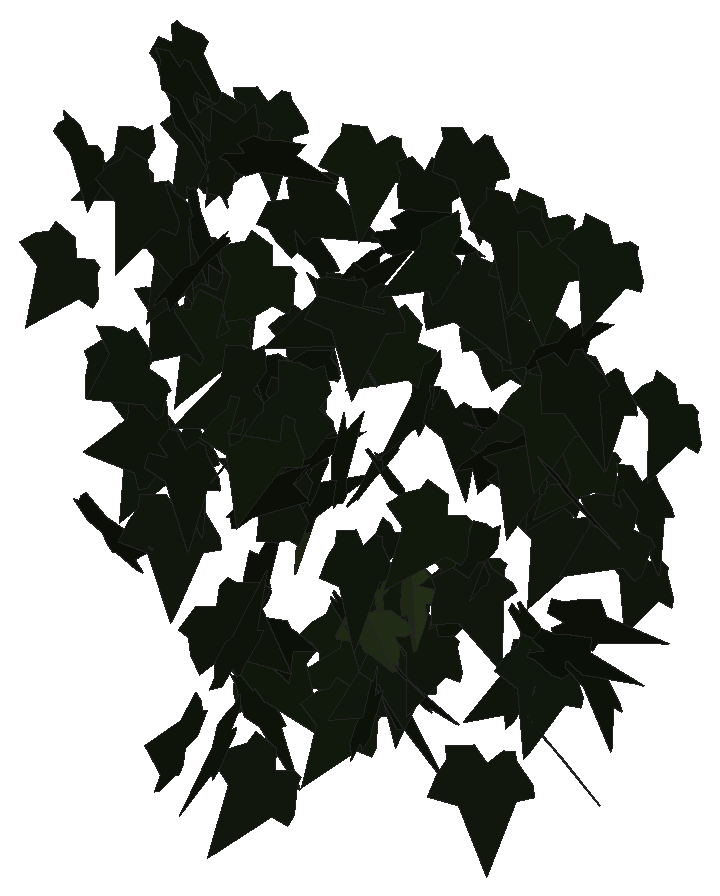
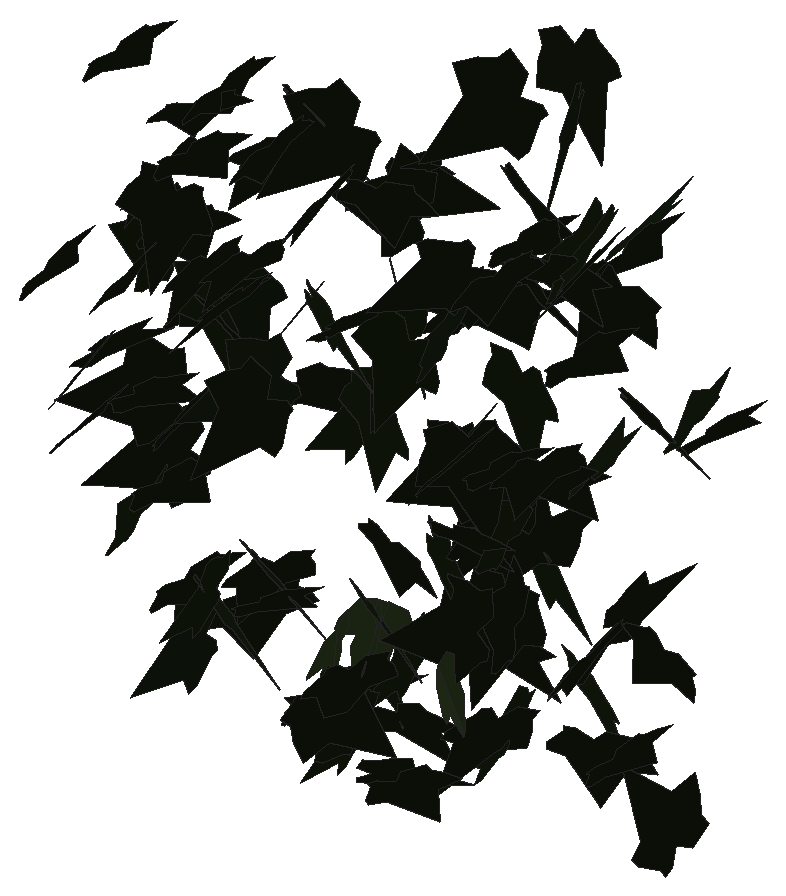
# SketchUp Ruby script. Lengths in inches.
U = 1.inch
M = Sketchup.active_model
def pt(a) = Geom::Point3d.new(a.map { |v| v * U })
def face(e, loops, mat)
  f = e.add_face(loops[0].map { |a| pt(a) })
  loops[1..].each { |l| e.add_face(l.map { |a| pt(a) }).erase! }
  f.material = f.back_material = mat if mat
  f
end
# faces: each face lists its corners as indices into pts; further lists are holes
def faces(e, pts, list, mat = nil) = list.each { |f| face(e, (f[0].is_a?(Array) ? f : [f]).map { |l| l.map { |i| pts[i] } }, mat) }
# xy, xz, yz: faces in a plane at the given z, y or x. An outline is a flat list of corners, or four numbers for a rectangle; further outlines are holes
def ring(l) = l.size == 4 ? [[l[0], l[1]], [l[2], l[1]], [l[2], l[3]], [l[0], l[3]]] : l.each_slice(2).to_a
def flat(e, list, mat, &to3) = list.each { |f| face(e, (f[0].is_a?(Array) ? f : [f]).map { |l| ring(l).map { |u, v| to3.(u, v) } }, mat) }
def xy(e, z, list, mat = nil) = flat(e, list, mat) { |x, y| [x, y, z] }
def xz(e, y, list, mat = nil) = flat(e, list, mat) { |x, z| [x, y, z] }
def yz(e, x, list, mat = nil) = flat(e, list, mat) { |y, z| [x, y, z] }
def lines(e, pts, list) = list.each { |a, b| e.add_line(pt(pts[a]), pt(pts[b])) }
# prism: a flat outline (further loops are holes) pulled along v
def prism(e, loops, v, mat = nil)
  f = face(e, loops, mat); d = Geom::Vector3d.new(v.map { |x| x * U })
  f.pushpull(f.normal.samedirection?(d) ? d.length : -d.length)
end
def box(e, o, s, mat = nil) = prism(e, [[o, [o[0] + s[0], o[1], o[2]], [o[0] + s[0], o[1] + s[1], o[2]], [o[0], o[1] + s[1], o[2]]]], [0, 0, s[2]], mat)
def at(x, y, z, deg = 0) = Geom::Transformation.translation(pt([x, y, z])) * Geom::Transformation.rotation(ORIGIN, Z_AXIS, deg.degrees)
def axes(o, x, y, z) = Geom::Transformation.new([*x, 0, *y, 0, *z, 0, *pt(o).to_a, 1])
def part(name) = M.definitions.add(name)
# library, detail: a bought-in or finely detailed component or shape, given as its bounding box
def library(name, o, s) = part(name).tap { |d| box(d.entities, o, s) }
def detail(e, o, s) = box(e.add_group.entities, o, s)
def put(e, d, t, mat = nil) = e.add_instance(d, t).tap { |i| i.material = mat if mat }
def group(e, t, mat = nil) = e.add_group.tap { |g| g.transformation = t; g.material = mat if mat }.entities
root = M.entities
M.materials.add("efeu1").color = [18, 25, 13]
M.materials.add("efeu2").color = [43, 57, 29]
c1 = part("ivyleaf_9")
p = [[1.54,2.16,1.25],[1.36,2.04,1.19],[-0.21,0.99,0.68],[-0.71,1.11,0.82],[-0.85,0.86,0.67],[-0.8,0.17,0.21],
  [-0.9,-0.01,0.1],[-0.67,-0.16,-0.02],[-0.08,-0.08,-0.05],[-0.03,-0.6,-0.4],[0.65,-0.88,-0.66],[0.83,-0.6,-0.49],
  [1.29,-0.42,-0.43],[1.8125,-0.07,-0.26],[1.21,0.44,0.15]]
faces(c1.entities,p,[[0,1,2,3,4,5,6,7,8,9,10,11,12,13,14]],"efeu1")
c2 = part("ivyleaf_10")
p = [[0,0.5,-0.03],[-0.0625,2.02,-0.43],[-0.19,2.01,-0.46],[-0.54,1.05,-0.29],[-0.52,0.625,-0.18],[-0.83,0.76,-0.28],
  [-1.16,0.64,-0.33],[-1.15,0.33,-0.24],[-0.77,-0.39,0.02],[-0.3,-0.51,0.16],[0.04,-0.48,0.23],[-0.02,2.01,-0.4375],
  [-0.06,2.01,-0.43],[0.04,-0.49,0.23],[0.67,-0.49,0.14],[1.38,0.36,-0.2],[1.375,0.51,-0.24],[0.81,0.65,-0.19],
  [0.62,0.59,-0.15],[0.6,1.09,-0.28],[0.5,1.23,-0.31]]
faces(c2.entities,p,[[0,1,2,3,4,5,6,7,8,9,10],[11,12,0,13,14,15,16,17,18,19,20]],"efeu2")
put(root,c1,axes([587.55,109.1,321.87],[-0.72826,-0.69552,1.1133],[-0.03534,-1.2623,-0.81172],[1.31223,-0.42,0.596]))
put(root,c1,axes([592.26,108.54,307.04],[-1.13952,0.73613,-0.62099],[0.53113,-0.32215,-1.35651],[-0.80338,-1.25712,-0.01601]))
put(root,c1,axes([590.89,108.03,328.35],[-0.38313,1.43362,-0.19459],[0.05066,-0.18788,-1.48393],[-1.44588,-0.38646,-0.00043]))
put(root,c1,axes([592.6,110.86,304.26],[-1.38279,-0.46875,-0.09816],[0.09636,0.02149,-1.46004],[0.46912,-1.3861,0.01056]))
put(root,c1,axes([591.54,109.78,309.39],[-0.99939,0.98729,-0.32059],[-0.27455,0.17776,1.40332],[1.00107,1.03439,0.06482]))
put(root,c1,axes([588.24,110.67,303.98],[-0.75989,1.06786,0.64427],[-0.34194,0.54714,-1.31017],[-1.19937,-0.83256,-0.03466]))
put(root,c1,axes([591.34,111.97,319.29],[-0.7287,-1.23215,-0.15341],[0.08749,0.12649,-1.43147],[1.23858,-0.73386,0.01085]))
put(root,c1,axes([588.37,111.2,328.16],[0.83103,-0.28067,-1.21153],[-1.10919,0.49166,-0.87473],[0.56239,1.38445,0.06503]))
put(root,c1,axes([590.68,111.88,320.77],[-1.35145,0.54253,0.34301],[-0.31812,0.12828,-1.45628],[-0.55748,-1.38838,-0.00051]))
put(root,c1,axes([589.53,111.39,310.48],[0.18456,-0.60274,-1.36473],[-0.14342,1.3616,-0.62075],[1.485,0.20641,0.10966]))
put(root,c1,axes([592.26,114.1,319.52],[-0.63385,-0.52593,1.13026],[-0.77577,-0.82614,-0.81947],[0.97584,-0.99837,0.08269]))
put(root,c1,axes([593.95,114.74,324.5],[-0.18122,-0.22106,-1.38757],[-0.20509,-1.37992,0.24662],[-1.39002,0.23242,0.14451]))
put(root,c1,axes([589.39,113.08,317.32],[-0.3047,1.34751,0.43821],[-0.13345,0.41894,-1.38106],[-1.41068,-0.33069,0.03599]))
put(root,c1,axes([593.32,114.23,316.73],[-0.3126,0.87701,1.11033],[0.23458,-1.08925,0.9264],[1.39534,0.3796,0.09301]))
put(root,c1,axes([582.71,115.36,325.89],[-0.29945,-1.32775,0.51119],[-0.09759,-0.50199,-1.36102],[1.4194,-0.31462,0.01427]))
put(root,c1,axes([593.94,115.03,324.8],[-0.41887,-1.33372,-0.2241],[0.06498,0.21449,-1.39795],[1.35085,-0.42387,-0.00225]))
put(root,c1,axes([589.25,114.15,308.42],[1.13339,0.72856,-0.4687],[-0.4165,-0.2185,-1.3468],[-0.75962,1.20687,0.03911]))
put(root,c1,axes([600.09,115.35,305.16],[-0.39374,-1.36873,-0.41622],[0.12123,0.39822,-1.42423],[1.42547,-0.41193,0.00615]))
put(root,c1,axes([597.43,115.9375,315.53],[-0.95399,-0.84654,0.23753],[-0.1992,-0.13328,-1.27503],[0.85637,-0.97404,-0.03197]))
put(root,c1,axes([588.62,114.41,329.87],[1.24553,0.5727,0.5016],[0.41004,0.30572,-1.36723],[-0.64145,1.30747,0.09999]))
put(root,c1,axes([587.9375,115.68,304.04],[0.88163,-1.14499,0.24024],[0.14961,-0.188,-1.44508],[1.16031,0.89423,0.00379]))
put(root,c1,axes([578.01,116.37,320.39],[-0.58756,-1.04687,0.60097],[-0.05788,-0.64318,-1.17699],[1.20572,-0.54103,0.23637]))
put(root,c1,axes([588.84,114.45,313.96],[0.54913,1.15124,0.63986],[0.28155,0.57463,-1.27548],[-1.28667,0.61707,-0.00601]))
put(root,c1,axes([603.56,115.99,319.02],[0.74567,-0.8168,0.88263],[0.68318,-0.56696,-1.10184],[0.98968,1.00679,0.09558]))
put(root,c1,axes([582.54,115.92,324.68],[-0.57246,-0.39235,-1.2628],[1.0282,0.7332,-0.69392],[0.8315,-1.17677,-0.01132]))
put(root,c1,axes([592.85,115.13,323.98],[0.32433,0.02009,1.35724],[0.90557,1.03631,-0.23174],[-1.01116,0.93454,0.2278]))
put(root,c1,axes([597.32,116.3,327.51],[-1.29482,0.49729,0.16789],[-0.15433,0.06643,-1.38701],[-0.50167,-1.30396,-0.00663]))
put(root,c1,axes([593.45,115.58,304.17],[0.27623,0.21539,1.30342],[-0.17185,1.32615,-0.18272],[-1.30987,-0.12856,0.29884]))
put(root,c1,axes([603.82,115.99,312.89],[1.01031,0.04668,0.96525],[0.95972,0.11508,-1.0101],[-0.11318,1.39255,0.05112]))
put(root,c1,axes([587.83,115.59,308.51],[-0.0046,-0.17837,1.46528],[0.44378,1.39734,0.1715],[-1.40781,0.44106,0.04927]))
put(root,c1,axes([591.84,117.12,304.04],[-1.14227,-0.52996,-0.07898],[0.07318,0.02994,-1.25922],[0.53079,-1.14461,0.00363]))
put(root,c1,axes([593.54,116.82,316.14],[1.12364,-0.80195,0.15563],[0.12309,-0.09543,-1.38045],[0.80759,1.13034,-0.00613]))
put(root,c1,axes([583.1,117.76,322.43],[-0.58454,-1.1918,0.42443],[-0.16387,-0.39228,-1.32721],[1.25447,-0.60658,0.0244]))
put(root,c1,axes([602.59,116.27,311.02],[1.18236,0.20201,0.70448],[0.69436,0.11895,-1.19949],[-0.23442,1.37117,0.00027]))
put(root,c1,axes([588.34,117.74,312.25],[-0.22292,-1.32039,-0.3434],[0.04805,-0.35533,1.33509],[-1.36346,0.20336,0.10319]))
put(root,c1,axes([580.83,118.08,312.22],[-0.37627,-0.3566,1.25662],[-0.67038,-1.06965,-0.50427],[1.1211,-0.75929,0.12022]))
put(root,c1,axes([591.93,117.54,311.33],[-0.92956,-0.39054,-0.96094],[0.96391,0.15142,-0.99397],[0.38317,-1.32837,0.16922]))
put(root,c1,axes([581.89,118.28,318.16],[-0.38795,-0.87853,0.97421],[0.22843,-1.04564,-0.85198],[1.29179,-0.07893,0.44323]))
put(root,c1,axes([596.47,117.87,319.15],[0.32534,-1.26749,0.32696],[0.08227,-0.31645,-1.30857],[1.30639,0.33557,0.00098]))
put(root,c1,axes([600.02,116.89,319.39],[-0.06645,1.4185,-0.5317],[-0.2088,-0.53571,-1.4031],[-1.50042,0.01173,0.21881]))
put(root,c1,axes([595.54,117.4375,320.15],[-1.17348,0.62304,-0.40212],[0.35495,-0.18896,-1.32862],[-0.65106,-1.22599,0.00043]))
put(root,c1,axes([602.68,117.45,323.47],[0.53871,-1.31162,-0.38333],[-0.12854,0.36157,-1.41783],[1.36043,0.55355,0.01783]))
put(root,c1,axes([587.51,116.96,305.2],[0.19302,-0.92808,-1.03853],[-0.00055,1.0484,-0.937],[1.39279,0.12903,0.14355]))
put(root,c1,axes([593.54,116.34,315.9],[-0.12957,1.16395,0.73041],[-0.21588,0.7073,-1.16542],[-1.35709,-0.22364,0.11566]))
put(root,c1,axes([600.1875,118.14,318.95],[-0.45765,-1.36902,0.17153],[0.08503,-0.20836,-1.43612],[1.3771,-0.4421,0.14567]))
put(root,c1,axes([601.68,117.89,321.54],[-0.60736,-1.15631,-0.13362],[0.06776,0.11534,-1.3061],[1.16203,-0.61109,0.00632]))
put(root,c1,axes([597.24,117.22,325.93],[0.05499,-0.99872,-0.93345],[0.28832,0.92166,-0.96912],[1.33627,-0.15776,0.24751]))
put(root,c1,axes([590.11,117.84,322.08],[0.84233,-1.06892,0.55335],[0.3445,-0.43303,-1.36092],[1.1533,0.91005,0.00238]))
put(root,c1,axes([586.02,116.68,327.28],[-0.18204,0.63679,1.31638],[-0.85793,1.02774,-0.6158],[-1.1842,-0.84247,0.24378]))
put(root,c1,axes([589.3,116.3,314.92],[0.56764,0.58795,1.0697],[0.56353,0.92024,-0.80484],[-1.08277,0.78717,0.14191]))
put(root,c1,axes([594.66,116.65,327.51],[1.11598,0.7508,0.52686],[0.43876,0.29168,-1.34504],[-0.80547,1.19913,-0.0027]))
put(root,c1,axes([592.61,118.84,305.05],[-0.66064,-0.68803,0.88155],[-0.34399,-0.84921,-0.92058],[1.06404,-0.70172,0.24973]))
put(root,c2,axes([592.36,117.62,308.11],[-1.11381,-0.5065,-0.34144],[0.30096,0.16288,-1.22335],[0.53155,-1.15353,-0.02281]))
put(root,c1,axes([602.91,118.59,309.26],[0.45181,-1.18045,0.63929],[0.27655,-0.57821,-1.26312],[1.31365,0.52772,0.04604]))
put(root,c1,axes([582.25,118.56,327.39],[0.76171,-1.13179,0.51572],[0.2797,-0.43338,-1.36421],[1.2119,0.81139,-0.00929]))
put(root,c1,axes([598.91,118.78,328.65],[-0.08384,-1.38207,0.15317],[-0.0065,-0.15306,-1.38461],[1.39051,-0.08404,0.00277]))
put(root,c1,axes([587.95,117.7,317.58],[0.89105,-0.72957,-0.67448],[-0.30746,0.65904,-1.11906],[0.94481,0.90252,0.27194]))
put(root,c1,axes([593.32,119.13,320.68],[-0.82787,-0.73034,0.72215],[-0.20952,-0.78794,-1.03707],[1.00548,-0.76552,0.37848]))
put(root,c1,axes([600.6,117.94,318.2],[-1.0696,0.60869,0.83669],[-0.7462,0.37983,-1.23024],[-0.71675,-1.30377,0.03221]))
put(root,c1,axes([604.35,119.23,315.89],[-0.76304,-0.75243,0.82337],[-0.29466,-0.82617,-1.02807],[1.07576,-0.76,0.30241]))
put(root,c1,axes([603.54,119.08,328.7],[-0.36808,-1.28406,0.32494],[-0.02164,-0.33138,-1.33402],[1.32436,-0.3623,0.06851]))
put(root,c1,axes([600.18,118.77,327.49],[-0.35947,-1.24355,-0.26908],[0.32621,0.18018,-1.26853],[1.2298,-0.41129,0.25784]))
put(root,c1,axes([600.25,117.9,319.53],[-0.53721,1.35212,0.05077],[-0.0718,0.02606,-1.45382],[-1.35117,-0.53898,0.05707]))
put(root,c1,axes([584.49,119.3,327.49],[-0.52444,-1.14335,0.3608],[-0.0584,-0.36897,-1.25416],[1.19751,-0.51872,0.09684]))
put(root,c1,axes([590.29,118.28,307.76],[1.09488,-0.57027,-0.27413],[-0.22887,0.15384,-1.23413],[0.58989,1.11815,0.02998]))
put(root,c1,axes([583.36,119.25,318.02],[-0.99314,-0.87565,-0.0172],[0.01233,0.01202,-1.32404],[0.87573,-0.99322,-0.00086]))
put(root,c1,axes([592.65,119.31,305.77],[-0.11975,-1.24972,0.09422],[0.01096,-0.09569,-1.25528],[1.25322,-0.11858,0.01998]))
put(root,c1,axes([599.95,119.54,307.96],[-0.3404,-1.32051,0.19637],[-0.05493,-0.18863,-1.36367],[1.3339,-0.34475,-0.00604]))
put(root,c1,axes([583.03,119.25,326.95],[-1.20353,-0.51015,-0.24264],[0.21327,0.11847,-1.30694],[0.52311,-1.22202,-0.02541]))
put(root,c1,axes([581.24,119.53,311.19],[0.16256,-1.39094,0.187],[-0.00787,-0.18915,-1.40009],[1.40343,0.16005,-0.02951]))
put(root,c1,axes([592.32,118.83,304.38],[1.13985,-0.84957,-0.16786],[-0.13417,0.10087,-1.42163],[0.85553,1.14772,0.00069]))
put(root,c1,axes([588.46,119.22,313.35],[-1.02388,0.55738,-0.66076],[0.56683,-0.34044,-1.16551],[-0.65267,-1.17005,0.02435]))
put(root,c1,axes([587.29,118.76,317.82],[0.3044,1.14447,-0.73418],[-0.19248,-0.7085,-1.18425],[-1.34602,0.36014,0.00332]))
put(root,c1,axes([599.6875,118.93,305.4],[1.33679,-0.52591,-0.02799],[-0.02572,0.01108,-1.43652],[0.52603,1.33704,0.00089]))
put(root,c1,axes([575.78,120.01,323.23],[0.11473,-1.05693,0.82305],[0.28798,-0.78729,-1.05115],[1.30828,0.26599,0.1592]))
put(root,c1,axes([599.15,119.09,307.41],[-1.23794,0.77954,0.0722],[-0.06097,0.03866,-1.46294],[-0.7805,-1.23944,-0.00023]))
put(root,c1,axes([584.59,119.95,315.25],[0.38279,-0.93172,0.93945],[0.47549,-0.81577,-1.00281],[1.23474,0.603,0.09492]))
put(root,c1,axes([580.875,119.71,328.61],[0.64598,-1.18876,0.24908],[0.10487,-0.22647,-1.35284],[1.21004,0.65425,-0.01572]))
put(root,c1,axes([592.2,119.61,304.6],[0.67217,-0.66735,0.87858],[0.76372,-0.46103,-0.93449],[0.79624,1.00557,0.15464]))
put(root,c1,axes([580.66,119.71,307.95],[-0.90836,-0.84881,-0.71897],[0.53268,0.48297,-1.24319],[0.97655,-1.05299,0.00935]))
put(root,c2,axes([591.02,119.57,309.02],[-0.50807,1.01692,-0.54611],[0.18072,-0.51923,-1.13501],[-1.14005,-0.53551,0.06346]))
put(root,c1,axes([580.8,119.85,311.62],[0.38032,-1.35861,-0.05097],[-0.01482,0.04878,-1.41084],[1.35949,0.38061,-0.00112]))
put(root,c1,axes([587.23,118.99,325.21],[0.20841,-0.07674,-1.38118],[0.43743,1.32875,-0.00782],[1.31233,-0.43072,0.22195]))
put(root,c1,axes([591.46,119.32,309.7],[-0.80626,0.80915,0.54487],[-0.37539,0.3951,-1.14221],[-0.90039,-0.88929,-0.0117]))
put(root,c1,axes([600.98,118.96,323.51],[0.37118,1.26574,0.06994],[0.0254,0.06543,-1.31903],[-1.26742,0.372,-0.00595]))
put(root,c1,axes([595.66,119.83,310.18],[-0.00235,-1.10531,-0.68086],[0.12469,0.67752,-1.10032],[1.29218,-0.06739,0.10494]))
put(root,c1,axes([587.23,120.18,322.85],[0.70942,-1.03812,0.32015],[0.16949,-0.27192,-1.2573],[1.07306,0.72927,-0.01307]))
put(root,c1,axes([576.45,120.32,305.54],[0.19082,-0.55782,1.32464],[1.00155,-0.90682,-0.52615],[1.0309,0.98426,0.26598]))
put(root,c1,axes([603.96,120.79,313.53],[-0.20286,-1.13699,0.59075],[0.09261,-0.60956,-1.14138],[1.27795,-0.13631,0.17649]))
put(root,c1,axes([596.04,119.21,317.63],[1.29152,0.15252,0.42652],[0.3517,0.47451,-1.23465],[-0.28546,1.27467,0.40858]))
put(root,c1,axes([586.73,120.91,317.85],[-0.22061,-1.11031,0.60959],[0.08842,-0.63076,-1.11686],[1.26355,-0.14971,0.18459]))
put(root,c1,axes([590.26,120.42,328.04],[-0.89237,-0.80246,-0.52832],[0.41651,0.32666,-1.19967],[0.86579,-0.98425,0.03258]))
put(root,c1,axes([592.98,120.97,306.12],[-0.28943,-1.1448,0.445],[-0.05561,-0.44451,-1.1797],[1.22699,-0.29019,0.0515]))
put(root,c1,axes([586.27,120.8,315.33],[-1.14536,-0.51639,-0.17128],[0.25595,-0.15916,-1.23167],[0.48009,-1.14711,0.248]))
put(root,c1,axes([578.36,120.26,323.17],[-1.20804,0.44614,0.26944],[-0.2607,0.0717,-1.28759],[-0.4513,-1.23564,0.02257]))
put(root,c1,axes([596.49,120.24,323],[0.27773,-1.12082,-0.60678],[0.09054,0.6368,-1.13483],[1.2713,0.1995,0.21337]))
put(root,c1,axes([589.98,120.88,303.87],[-0.99225,-0.08441,0.75828],[-0.7014,-0.38861,-0.96109],[0.30024,-1.18682,0.26077]))
put(root,c2,axes([592.29,120.42,308.56],[-0.16772,1.21082,-0.34158],[0.03723,-0.33967,-1.22234],[-1.25753,-0.17155,0.00937]))
put(root,c1,axes([586.59,119.42,310.35],[0.41624,0.36053,1.25445],[0.91825,0.85487,-0.55037],[-0.92761,1.00802,0.01808]))
put(root,c1,axes([576.67,120.7,313.62],[-0.42267,-0.47061,-1.11979],[1.06635,0.42397,-0.58068],[0.58163,-1.1193,0.25087]))
put(root,c1,axes([598.43,121.27,327.15],[-0.57454,-1.19737,0.16548],[-0.01944,-0.17404,-1.32684],[1.2086,-0.572,0.05732]))
put(root,c1,axes([598.88,121.51,315.78],[-0.21406,-1.01009,0.80251],[-0.05448,-0.80568,-1.02861],[1.28893,-0.2018,0.0898]))
put(root,c1,axes([592.3125,121.14,306.37],[-0.17685,0.48602,-1.27275],[0.12482,-1.27225,-0.50317],[-1.35666,-0.18041,0.11962]))
put(root,c1,axes([582.41,120.74,319.51],[-0.06277,-1.19796,-0.55241],[0.10962,0.54639,-1.19735],[1.31463,-0.10276,0.07347]))
put(root,c1,axes([601.43,121.24,320.96],[0.15194,-1.31759,0.25893],[0.03955,-0.25607,-1.32629],[1.34221,0.1567,0.00978]))
put(root,c1,axes([598.09,120.69,322.49],[0.33405,-1.10321,-0.59625],[-0.10245,0.59097,-1.15084],[1.24983,0.3433,0.06503]))
put(root,c1,axes([595.64,120.6,310.7],[-1.05255,0.74505,0.34822],[-0.31629,0.15534,-1.28843],[-0.75915,-1.09772,0.05401]))
put(root,c1,axes([597.69,120.74,308.84],[1.01017,-0.77261,-0.12133],[-0.09254,0.07872,-1.27174],[0.77658,1.01438,0.00628]))
put(root,c1,axes([592.375,121.07,327.26],[0.47756,-1.25207,-0.18062],[-0.05345,0.17292,-1.34],[1.2639,0.4804,0.01158]))
put(root,c1,axes([596.71,120.49,321.52],[0.71171,-0.8815,-0.68058],[-0.05026,0.78144,-1.0647],[1.11252,0.59922,0.38728]))
put(root,c1,axes([579.89,120.57,329.06],[0.80119,-0.87049,-0.63857],[-0.20792,0.65591,-1.15498],[1.05938,0.78706,0.25626]))
put(root,c1,axes([599.17,121.83,313.32],[-0.59329,-1.21783,0.29633],[-0.0894,-0.28591,-1.35396],[1.25018,-0.59839,0.04381]))
put(root,c1,axes([594.53,121.84,309.93],[-0.78929,-0.92994,0.32794],[0.03034,-0.44276,-1.18252],[0.98561,-0.73109,0.29902]))
put(root,c1,axes([603.22,121.48,316.55],[0.3925,-1.23269,0.17099],[0.04223,-0.166,-1.29363],[1.24378,0.39464,-0.01004]))
put(root,c2,axes([586.33,121.34,309.32],[0.43221,-1.13409,0.29773],[0.10846,-0.27729,-1.21366],[1.16749,0.4456,0.00252]))
put(root,c1,axes([588.3,121.63,304.42],[-0.78025,-0.97691,-0.0115],[0.00794,0.00838,-1.25025],[0.97694,-0.78029,0.00097]))
put(root,c1,axes([604.57,121.96,320.46],[-0.18786,-1.15985,0.59786],[-0.07377,-0.59361,-1.1748],[1.30278,-0.20086,0.01968]))
put(root,c1,axes([594.41,121.57,328.97],[0.12089,-1.33246,-0.04934],[-0.01964,0.04776,-1.33785],[1.33323,0.12152,-0.01523]))
put(root,c1,axes([595.59,120.48,317.375],[1.30327,0.37645,0.03702],[0.03553,0.0104,-1.35655],[-0.37659,1.30376,0.00013]))
put(root,c1,axes([590.88,121.29,308.04],[-0.09591,-1.18698,-0.55787],[0.03217,0.55706,-1.19079],[1.31115,-0.10049,-0.01159]))
put(root,c1,axes([577.82,122.04,309.32],[-0.4312,-1.17383,0.45924],[-0.08949,-0.45564,-1.24864],[1.25729,-0.43501,0.06863]))
put(root,c1,axes([600.2,122.05,316.79],[-0.81897,-0.913,0.44209],[-0.13702,-0.46342,-1.21086],[1.0051,-0.80709,0.19515]))
put(root,c1,axes([583.54,122.0625,319.46],[-0.73509,-0.97402,0.41867],[-0.10992,-0.4367,-1.20895],[1.05447,-0.72453,0.16584]))
put(root,c1,axes([583.84,121.6,327.19],[-0.05818,-1.31597,-0.24903],[-0.01606,0.24993,-1.31699],[1.33923,-0.05417,-0.02661]))
put(root,c1,axes([589.08,120.1875,321.96],[0.30327,1.23705,0.48871],[0.02075,0.49679,-1.27039],[-1.32993,0.28984,0.09162]))
